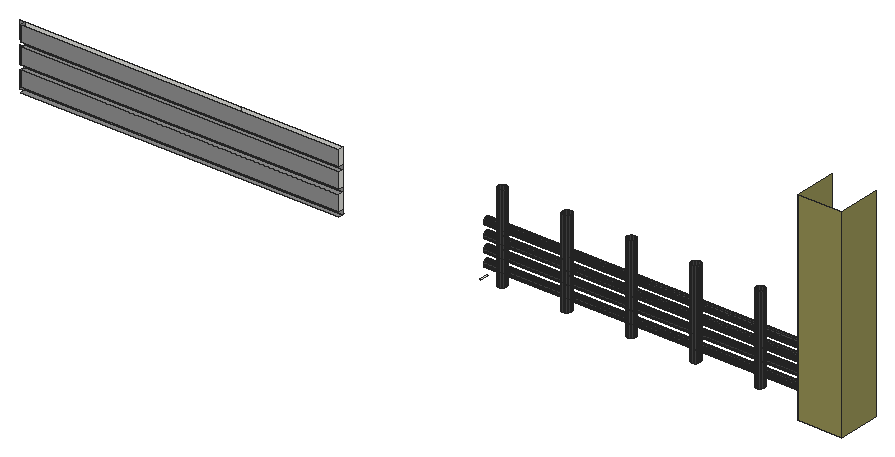
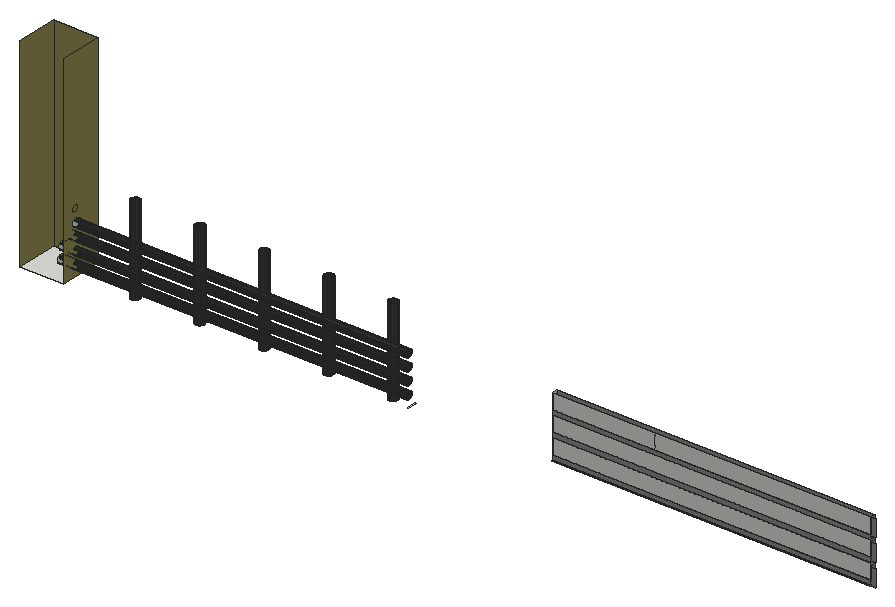
# SketchUp Ruby script. Lengths in inches.
U = 1.inch
M = Sketchup.active_model
def pt(a) = Geom::Point3d.new(a.map { |v| v * U })
def face(e, loops, mat)
  f = e.add_face(loops[0].map { |a| pt(a) })
  loops[1..].each { |l| e.add_face(l.map { |a| pt(a) }).erase! }
  f.material = f.back_material = mat if mat
  f
end
# faces: each face lists its corners as indices into pts; further lists are holes
def faces(e, pts, list, mat = nil) = list.each { |f| face(e, (f[0].is_a?(Array) ? f : [f]).map { |l| l.map { |i| pts[i] } }, mat) }
# xy, xz, yz: faces in a plane at the given z, y or x. An outline is a flat list of corners, or four numbers for a rectangle; further outlines are holes
def ring(l) = l.size == 4 ? [[l[0], l[1]], [l[2], l[1]], [l[2], l[3]], [l[0], l[3]]] : l.each_slice(2).to_a
def flat(e, list, mat, &to3) = list.each { |f| face(e, (f[0].is_a?(Array) ? f : [f]).map { |l| ring(l).map { |u, v| to3.(u, v) } }, mat) }
def xy(e, z, list, mat = nil) = flat(e, list, mat) { |x, y| [x, y, z] }
def xz(e, y, list, mat = nil) = flat(e, list, mat) { |x, z| [x, y, z] }
def yz(e, x, list, mat = nil) = flat(e, list, mat) { |y, z| [x, y, z] }
def lines(e, pts, list) = list.each { |a, b| e.add_line(pt(pts[a]), pt(pts[b])) }
# prism: a flat outline (further loops are holes) pulled along v
def prism(e, loops, v, mat = nil)
  f = face(e, loops, mat); d = Geom::Vector3d.new(v.map { |x| x * U })
  f.pushpull(f.normal.samedirection?(d) ? d.length : -d.length)
end
def box(e, o, s, mat = nil) = prism(e, [[o, [o[0] + s[0], o[1], o[2]], [o[0] + s[0], o[1] + s[1], o[2]], [o[0], o[1] + s[1], o[2]]]], [0, 0, s[2]], mat)
def at(x, y, z, deg = 0) = Geom::Transformation.translation(pt([x, y, z])) * Geom::Transformation.rotation(ORIGIN, Z_AXIS, deg.degrees)
def axes(o, x, y, z) = Geom::Transformation.new([*x, 0, *y, 0, *z, 0, *pt(o).to_a, 1])
def part(name) = M.definitions.add(name)
# library, detail: a bought-in or finely detailed component or shape, given as its bounding box
def library(name, o, s) = part(name).tap { |d| box(d.entities, o, s) }
def detail(e, o, s) = box(e.add_group.entities, o, s)
def put(e, d, t, mat = nil) = e.add_instance(d, t).tap { |i| i.material = mat if mat }
def group(e, t, mat = nil) = e.add_group.tap { |g| g.transformation = t; g.material = mat if mat }.entities
root = M.entities
M.materials.add("[0057_DarkKhaki]").color = [150, 145, 85]
M.materials.add("[0137_Black]").color = [71, 71, 71]
M.materials.add("[Color M05]").color = [145, 145, 145]
xy(root,379.43,[[[484.5625,1.0625,510.6875,26.4375],[488.89,12.9375,489.58,13.03,490.23,13.3,490.79,13.72,491.21,14.28,491.48,14.93,491.57,15.625,491.48,16.32,491.22,16.97,490.79,17.53,490.23,17.95,489.58,18.22,488.89,18.3125,488.19,18.22,487.54,17.95,486.99,17.53,486.56,16.97,486.29,16.32,486.2,15.625,486.29,14.93,486.56,14.28,486.99,13.73,487.54,13.3,488.19,13.03]],[488.89,12.9375,488.19,13.03,487.54,13.3,486.99,13.73,486.56,14.28,486.29,14.93,486.2,15.625,486.29,16.32,486.56,16.97,486.99,17.53,487.54,17.95,488.19,18.22,488.89,18.3125,489.58,18.22,490.23,17.95,490.79,17.53,491.22,16.97,491.48,16.32,491.57,15.625,491.48,14.93,491.21,14.28,490.79,13.72,490.23,13.3,489.58,13.03],[286.17,13.0625,286.99,18.1875]])
xy(root,381.65,[[11.875,18.1875,200.79,19]])
xy(root,381.65,[[11.875,15.1875,200.79,18.1875]],"[Color M05]")
xy(root,384.55,[[11.875,15.1875,200.79,18.1875]],"[Color M05]")
xy(root,393.65,[[11.875,15.1875,200.79,18.1875]],"[Color M05]")
xy(root,396.55,[[11.875,15.1875,200.79,18.1875]],"[Color M05]")
xy(root,405.65,[[11.875,15.1875,200.79,18.1875]],"[Color M05]")
xy(root,408.55,[[11.875,15.1875,200.79,18.1875]],"[Color M05]")
xz(root,1.0625,[[484.5625,379.43,510.6875,499.43]],"[0057_DarkKhaki]")
xz(root,15.1875,[[11.875,384.55,200.79,393.65],[11.875,396.55,200.79,405.65],[11.875,408.55,200.79,417.65]],"[Color M05]")
xz(root,18.1875,[[11.875,384.55,200.79,393.65],[11.875,396.55,200.79,405.65],[11.875,408.55,139.9375,417.65],[139.9375,408.55,200.79,417.65]])
xz(root,18.1875,[[8.875,381.32,11.875,391.4],[11.875,381.65,200.79,384.55],[11.875,393.65,200.79,396.55],[8.875,394.44,11.875,404.53],[11.875,405.65,200.79,408.55],
  [8.875,407.57,11.875,417.65]],"[Color M05]")
yz(root,11.875,[[18.1875,381.32,19,381.65]])
yz(root,11.875,[[15.1875,384.55,18.1875,391.4],[15.1875,391.4,18.1875,393.65],[15.1875,396.55,18.1875,404.53],[15.1875,404.53,18.1875,405.65],[15.1875,408.55,18.1875,417.65]],"[Color M05]")
yz(root,200.79,[[15.1875,384.55,18.1875,393.65],[15.1875,396.55,18.1875,405.65],[15.1875,408.55,18.1875,417.65]])
yz(root,484.11,[[18.04,406.36,18.63,406.44,19.17,406.66,19.64,407.02,19.99,407.49,20.22,408.03,20.29,408.61,20.22,409.2,19.99,409.74,19.64,410.2,19.17,410.5625,18.63,410.79,18.04,410.86,17.46,410.79,16.92,410.5625,16.45,410.2,16.1,409.74,15.87,409.2,15.79,408.61,15.87,408.03,16.1,407.49,16.45,407.02,16.92,406.66,17.46,406.44]])
yz(root,484.5625,[[[1.0625,379.43,26.4375,499.43],[18.04,413.86,18.63,413.94,19.17,414.16,19.64,414.52,19.99,414.99,20.22,415.53,20.29,416.11,20.22,416.7,19.99,417.24,19.64,417.7,19.17,418.0625,18.63,418.29,18.04,418.36,17.46,418.29,16.92,418.0625,16.45,417.7,16.1,417.24,15.87,416.7,15.79,416.11,15.87,415.53,16.1,414.99,16.45,414.52,16.92,414.16,17.46,413.94]]],"[0057_DarkKhaki]")
yz(root,487.23,[[18.04,398.86,18.63,398.94,19.17,399.16,19.64,399.52,19.99,399.99,20.22,400.53,20.29,401.11,20.22,401.7,19.99,402.24,19.64,402.7,19.17,403.0625,18.63,403.29,18.04,403.36,17.46,403.29,16.92,403.0625,16.45,402.7,16.1,402.24,15.87,401.7,15.79,401.11,15.87,400.53,16.1,399.99,16.45,399.52,16.92,399.16,17.46,398.94]])
yz(root,492.3,[[18.04,391.36,18.63,391.44,19.17,391.66,19.64,392.02,19.99,392.49,20.22,393.03,20.29,393.61,20.22,394.2,19.99,394.74,19.64,395.2,19.17,395.5625,18.63,395.79,18.04,395.86,17.46,395.79,16.92,395.5625,16.45,395.2,16.1,394.74,15.87,394.2,15.79,393.61,15.87,393.03,16.1,392.49,16.45,392.02,16.92,391.66,17.46,391.44]])
yz(root,492.98,[[18.04,383.86,18.63,383.94,19.17,384.16,19.64,384.52,19.99,384.99,20.22,385.53,20.29,386.11,20.22,386.7,19.99,387.24,19.64,387.7,19.17,388.0625,18.63,388.29,18.04,388.36,17.46,388.29,16.92,388.0625,16.45,387.7,16.1,387.24,15.87,386.7,15.79,386.11,15.87,385.53,16.1,384.99,16.45,384.52,16.92,384.16,17.46,383.94]])
yz(root,510.6875,[[1.0625,379.43,26.4375,499.43]],"[0057_DarkKhaki]")
p = [[296.94,13.03,379.43],[297.64,12.9375,379.43],[297.64,12.9375,431.18],[296.94,13.03,431.18],[298.33,13.03,379.43],[298.33,13.03,431.18],
  [335.19,13.03,379.43],[335.89,12.9375,379.43],[335.89,12.9375,431.18],[335.19,13.03,431.18],[336.58,13.03,379.43],[336.58,13.03,431.18],
  [373.44,13.03,379.43],[374.14,12.9375,379.43],[374.14,12.9375,431.18],[373.44,13.03,431.18],[374.83,13.03,379.43],[374.83,13.03,431.18],
  [411.69,13.03,379.43],[412.39,12.9375,379.43],[412.39,12.9375,431.18],[411.69,13.03,431.18],[413.08,13.03,379.43],[413.08,13.03,431.18],
  [449.94,13.03,379.43],[450.64,12.9375,379.43],[450.64,12.9375,431.18],[449.94,13.03,431.18],[451.33,13.03,379.43],[451.33,13.03,431.18],
  [296.29,13.3,379.43],[296.29,13.3,431.18],[298.98,13.3,379.43],[298.98,13.3,431.18],[334.54,13.3,379.43],[334.54,13.3,431.18],
  [337.23,13.3,379.43],[337.23,13.3,431.18],[372.79,13.3,379.43],[372.79,13.3,431.18],[375.48,13.3,379.43],[375.48,13.3,431.18],
  [411.04,13.3,379.43],[411.04,13.3,431.18],[413.73,13.3,379.43],[413.73,13.3,431.18],[449.29,13.3,379.43],[449.29,13.3,431.18],
  [451.98,13.3,379.43],[451.98,13.3,431.18],[295.74,13.73,379.43],[295.74,13.73,431.18],[299.54,13.72,379.43],[299.54,13.72,431.18],
  [333.99,13.73,379.43],[333.99,13.73,431.18],[337.79,13.72,379.43],[337.79,13.72,431.18],[372.24,13.73,379.43],[372.24,13.73,431.18],
  [376.04,13.72,379.43],[376.04,13.72,431.18],[410.49,13.73,379.43],[410.49,13.73,431.18],[414.29,13.72,379.43],[414.29,13.72,431.18],
  [448.74,13.73,379.43],[448.74,13.73,431.18],[452.54,13.72,379.43],[452.54,13.72,431.18],[295.31,14.28,379.43],[295.31,14.28,431.18],
  [299.96,14.28,379.43],[299.96,14.28,431.18],[333.56,14.28,379.43],[333.56,14.28,431.18],[338.21,14.28,379.43],[338.21,14.28,431.18],
  [371.81,14.28,379.43],[371.81,14.28,431.18],[376.46,14.28,379.43],[376.46,14.28,431.18],[410.06,14.28,379.43],[410.06,14.28,431.18],
  [414.71,14.28,379.43],[414.71,14.28,431.18],[448.31,14.28,379.43],[448.31,14.28,431.18],[452.96,14.28,379.43],[452.96,14.28,431.18],
  [295.04,14.93,379.43],[295.04,14.93,431.18],[300.23,14.93,379.43],[300.23,14.93,431.18],[333.29,14.93,379.43],[333.29,14.93,431.18],
  [338.48,14.93,379.43],[338.48,14.93,431.18],[371.54,14.93,379.43],[371.54,14.93,431.18],[376.73,14.93,379.43],[376.73,14.93,431.18],
  [409.79,14.93,379.43],[409.79,14.93,431.18],[414.98,14.93,379.43],[414.98,14.93,431.18],[448.04,14.93,379.43],[448.04,14.93,431.18],
  [453.23,14.93,379.43],[453.23,14.93,431.18],[294.95,15.625,379.43],[294.95,15.625,431.18],[300.32,15.625,379.43],[300.32,15.625,431.18],
  [333.2,15.625,379.43],[333.2,15.625,431.18],[338.57,15.625,379.43],[338.57,15.625,431.18],[371.45,15.625,379.43],[371.45,15.625,431.18],
  [376.82,15.625,379.43],[376.82,15.625,431.18],[409.7,15.625,379.43],[409.7,15.625,431.18],[415.07,15.625,379.43],[415.07,15.625,431.18],
  [447.95,15.625,379.43],[447.95,15.625,431.18],[453.32,15.625,379.43],[453.32,15.625,431.18],[295.04,16.32,379.43],[295.04,16.32,431.18],
  [300.23,16.32,379.43],[300.23,16.32,431.18],[333.29,16.32,379.43],[333.29,16.32,431.18],[338.48,16.32,379.43],[338.48,16.32,431.18],
  [371.54,16.32,379.43],[371.54,16.32,431.18],[376.73,16.32,379.43],[376.73,16.32,431.18],[409.79,16.32,379.43],[409.79,16.32,431.18],
  [414.98,16.32,379.43],[414.98,16.32,431.18],[448.04,16.32,379.43],[448.04,16.32,431.18],[453.23,16.32,379.43],[453.23,16.32,431.18],
  [295.31,16.97,379.43],[295.31,16.97,431.18],[299.97,16.97,379.43],[299.97,16.97,431.18],[333.56,16.97,379.43],[333.56,16.97,431.18],
  [338.22,16.97,379.43],[338.22,16.97,431.18],[371.81,16.97,379.43],[371.81,16.97,431.18],[376.47,16.97,379.43],[376.47,16.97,431.18],
  [410.06,16.97,379.43],[410.06,16.97,431.18],[414.72,16.97,379.43],[414.72,16.97,431.18],[448.31,16.97,379.43],[448.31,16.97,431.18],
  [452.97,16.97,379.43],[452.97,16.97,431.18],[295.74,17.53,379.43],[295.74,17.53,431.18],[299.54,17.53,379.43],[299.54,17.53,431.18],
  [333.99,17.53,379.43],[333.99,17.53,431.18],[337.79,17.53,379.43],[337.79,17.53,431.18],[372.24,17.53,379.43],[372.24,17.53,431.18],
  [376.04,17.53,379.43],[376.04,17.53,431.18],[410.49,17.53,379.43],[410.49,17.53,431.18],[414.29,17.53,379.43],[414.29,17.53,431.18],
  [448.74,17.53,379.43],[448.74,17.53,431.18],[452.54,17.53,379.43],[452.54,17.53,431.18],[296.29,17.95,379.43],[296.29,17.95,431.18],
  [298.98,17.95,379.43],[298.98,17.95,431.18],[334.54,17.95,379.43],[334.54,17.95,431.18],[337.23,17.95,379.43],[337.23,17.95,431.18],
  [372.79,17.95,379.43],[372.79,17.95,431.18],[375.48,17.95,379.43],[375.48,17.95,431.18],[411.04,17.95,379.43],[411.04,17.95,431.18],
  [413.73,17.95,379.43],[413.73,17.95,431.18],[449.29,17.95,379.43],[449.29,17.95,431.18],[451.98,17.95,379.43],[451.98,17.95,431.18],
  [296.94,18.22,379.43],[296.94,18.22,431.18],[298.33,18.22,379.43],[298.33,18.22,431.18],[335.19,18.22,379.43],[335.19,18.22,431.18],
  [336.58,18.22,379.43],[336.58,18.22,431.18],[373.44,18.22,379.43],[373.44,18.22,431.18],[374.83,18.22,379.43],[374.83,18.22,431.18],
  [411.69,18.22,379.43],[411.69,18.22,431.18],[413.08,18.22,379.43],[413.08,18.22,431.18],[449.94,18.22,379.43],[449.94,18.22,431.18],
  [451.33,18.22,379.43],[451.33,18.22,431.18],[297.64,18.3125,379.43],[297.64,18.3125,431.18],[335.89,18.3125,379.43],[335.89,18.3125,431.18],
  [374.14,18.3125,379.43],[374.14,18.3125,431.18],[412.39,18.3125,379.43],[412.39,18.3125,431.18],[450.64,18.3125,379.43],[450.64,18.3125,431.18],
  [286.17,16.92,384.16],[286.17,17.46,383.94],[492.98,17.46,383.94],[492.98,16.92,384.16],[286.17,18.04,383.86],[492.98,18.04,383.86],
  [286.17,18.63,383.94],[492.98,18.63,383.94],[286.17,19.17,384.16],[492.98,19.17,384.16],[286.17,16.45,384.52],[492.98,16.45,384.52],
  [286.17,19.64,384.52],[492.98,19.64,384.52],[286.17,16.1,384.99],[492.98,16.1,384.99],[286.17,19.99,384.99],[492.98,19.99,384.99],
  [286.17,15.87,385.53],[492.98,15.87,385.53],[286.17,15.79,386.11],[492.98,15.79,386.11],[286.17,15.87,386.7],[492.98,15.87,386.7],
  [286.17,16.1,387.24],[492.98,16.1,387.24],[286.17,16.45,387.7],[492.98,16.45,387.7],[286.17,19.99,387.24],[286.17,19.64,387.7],
  [492.98,19.64,387.7],[492.98,19.99,387.24],[286.17,16.92,388.0625],[492.98,16.92,388.0625],[286.17,19.17,388.0625],[492.98,19.17,388.0625],
  [286.17,17.46,388.29],[492.98,17.46,388.29],[286.17,18.63,388.29],[492.98,18.63,388.29],[286.17,18.04,388.36],[492.98,18.04,388.36],
  [286.17,16.92,391.66],[286.17,17.46,391.44],[492.3,17.46,391.44],[492.3,16.92,391.66],[286.17,18.04,391.36],[492.3,18.04,391.36],
  [286.17,18.63,391.44],[492.3,18.63,391.44],[286.17,19.17,391.66],[492.3,19.17,391.66],[286.17,16.45,392.02],[492.3,16.45,392.02],
  [286.17,19.64,392.02],[492.3,19.64,392.02],[286.17,16.1,392.49],[492.3,16.1,392.49],[286.17,19.99,392.49],[492.3,19.99,392.49],
  [286.17,15.87,393.03],[492.3,15.87,393.03],[286.17,15.79,393.61],[492.3,15.79,393.61],[286.17,15.87,394.2],[492.3,15.87,394.2],
  [286.17,16.1,394.74],[492.3,16.1,394.74],[286.17,16.45,395.2],[492.3,16.45,395.2],[286.17,16.92,395.5625],[492.3,16.92,395.5625],
  [286.17,19.64,395.2],[286.17,19.17,395.5625],[492.3,19.17,395.5625],[492.3,19.64,395.2],[286.17,17.46,395.79],[492.3,17.46,395.79],
  [286.17,18.63,395.79],[492.3,18.63,395.79],[286.17,18.04,395.86],[492.3,18.04,395.86],[286.17,16.92,399.16],[286.17,17.46,398.94],
  [487.23,17.46,398.94],[487.23,16.92,399.16],[286.17,18.04,398.86],[487.23,18.04,398.86],[286.17,18.63,398.94],[487.23,18.63,398.94],
  [286.17,19.17,399.16],[487.23,19.17,399.16],[286.17,16.45,399.52],[487.23,16.45,399.52],[286.17,19.64,399.52],[487.23,19.64,399.52],
  [286.17,16.1,399.99],[487.23,16.1,399.99],[286.17,15.87,400.53],[487.23,15.87,400.53],[286.17,15.79,401.11],[487.23,15.79,401.11],
  [286.17,15.87,401.7],[487.23,15.87,401.7],[286.17,16.1,402.24],[487.23,16.1,402.24],[286.17,16.45,402.7],[487.23,16.45,402.7],
  [286.17,16.92,403.0625],[487.23,16.92,403.0625],[286.17,19.64,402.7],[286.17,19.17,403.0625],[487.23,19.17,403.0625],[487.23,19.64,402.7],
  [286.17,17.46,403.29],[487.23,17.46,403.29],[286.17,18.63,403.29],[487.23,18.63,403.29],[286.17,18.04,403.36],[487.23,18.04,403.36],
  [286.17,16.92,406.66],[286.17,17.46,406.44],[484.11,17.46,406.44],[484.11,16.92,406.66],[286.17,18.04,406.36],[484.11,18.04,406.36],
  [286.17,18.63,406.44],[484.11,18.63,406.44],[286.17,19.17,406.66],[484.11,19.17,406.66],[286.17,16.45,407.02],[484.11,16.45,407.02],
  [286.17,19.64,407.02],[484.11,19.64,407.02],[286.17,16.1,407.49],[484.11,16.1,407.49],[286.17,15.87,408.03],[484.11,15.87,408.03],
  [286.17,15.79,408.61],[484.11,15.79,408.61],[286.17,15.87,409.2],[484.11,15.87,409.2],[286.17,16.1,409.74],[484.11,16.1,409.74],
  [286.17,16.45,410.2],[484.11,16.45,410.2],[286.17,16.92,410.5625],[484.11,16.92,410.5625],[286.17,19.64,410.2],[286.17,19.17,410.5625],
  [484.11,19.17,410.5625],[484.11,19.64,410.2],[286.17,17.46,410.79],[484.11,17.46,410.79],[286.17,18.63,410.79],[484.11,18.63,410.79],
  [286.17,18.04,410.86],[484.11,18.04,410.86],[284.41,1.0625,379.43],[284.05,1.0625,379.43],[285.29,1.0625,379.43],[286.99,1.0625,379.43],
  [11.875,19,381.65],[8.875,19,381.65]]
faces(root,p,[[0,1,2,3],[1,4,5,2],[6,7,8,9],[7,10,11,8],[12,13,14,15],[13,16,17,14],[18,19,20,21],[19,22,23,20],
  [24,25,26,27],[25,28,29,26],[30,0,3,31],[4,32,33,5],[34,6,9,35],[10,36,37,11],[38,12,15,39],[16,40,41,17],
  [42,18,21,43],[22,44,45,23],[46,24,27,47],[28,48,49,29],[50,30,31,51],[32,52,53,33],[54,34,35,55],[36,56,57,37],
  [58,38,39,59],[40,60,61,41],[62,42,43,63],[44,64,65,45],[66,46,47,67],[48,68,69,49],[70,50,51,71],[52,72,73,53],
  [74,54,55,75],[56,76,77,57],[78,58,59,79],[60,80,81,61],[82,62,63,83],[64,84,85,65],[86,66,67,87],[68,88,89,69],
  [90,70,71,91],[72,92,93,73],[94,74,75,95],[76,96,97,77],[98,78,79,99],[80,100,101,81],[102,82,83,103],[84,104,105,85],
  [106,86,87,107],[88,108,109,89],[110,90,91,111],[92,112,113,93],[114,94,95,115],[96,116,117,97],[118,98,99,119],[100,120,121,101],
  [122,102,103,123],[104,124,125,105],[126,106,107,127],[108,128,129,109],[130,110,111,131],[112,132,133,113],[134,114,115,135],[116,136,137,117],
  [138,118,119,139],[120,140,141,121],[142,122,123,143],[124,144,145,125],[146,126,127,147],[128,148,149,129],[150,130,131,151],[132,152,153,133],
  [154,134,135,155],[136,156,157,137],[158,138,139,159],[140,160,161,141],[162,142,143,163],[144,164,165,145],[166,146,147,167],[148,168,169,149],
  [170,150,151,171],[152,172,173,153],[174,154,155,175],[156,176,177,157],[178,158,159,179],[160,180,181,161],[182,162,163,183],[164,184,185,165],
  [186,166,167,187],[168,188,189,169],[190,170,171,191],[172,192,193,173],[194,174,175,195],[176,196,197,177],[198,178,179,199],[180,200,201,181],
  [202,182,183,203],[184,204,205,185],[206,186,187,207],[188,208,209,189],[210,190,191,211],[192,212,213,193],[214,194,195,215],[196,216,217,197],
  [218,198,199,219],[200,220,221,201],[222,202,203,223],[204,224,225,205],[226,206,207,227],[208,228,229,209],[230,210,211,231],[212,230,231,213],
  [232,214,215,233],[216,232,233,217],[234,218,219,235],[220,234,235,221],[236,222,223,237],[224,236,237,225],[238,226,227,239],[228,238,239,229],
  [240,241,242,243],[241,244,245,242],[244,246,247,245],[246,248,249,247],[250,240,243,251],[248,252,253,249],[254,250,251,255],[252,256,257,253],
  [258,254,255,259],[260,258,259,261],[262,260,261,263],[264,262,263,265],[266,264,265,267],[268,269,270,271],[272,266,267,273],[269,274,275,270],
  [276,272,273,277],[274,278,279,275],[280,276,277,281],[278,280,281,279],[282,283,284,285],[283,286,287,284],[286,288,289,287],[288,290,291,289],
  [292,282,285,293],[290,294,295,291],[296,292,293,297],[294,298,299,295],[300,296,297,301],[302,300,301,303],[304,302,303,305],[306,304,305,307],
  [308,306,307,309],[310,308,309,311],[312,313,314,315],[316,310,311,317],[313,318,319,314],[320,316,317,321],[318,320,321,319],[322,323,324,325],
  [323,326,327,324],[326,328,329,327],[328,330,331,329],[332,322,325,333],[330,334,335,331],[336,332,333,337],[338,336,337,339],[340,338,339,341],
  [342,340,341,343],[344,342,343,345],[346,344,345,347],[348,346,347,349],[350,351,352,353],[354,348,349,355],[351,356,357,352],[358,354,355,359],
  [356,358,359,357],[360,361,362,363],[361,364,365,362],[364,366,367,365],[366,368,369,367],[370,360,363,371],[368,372,373,369],[374,370,371,375],
  [376,374,375,377],[378,376,377,379],[380,378,379,381],[382,380,381,383],[384,382,383,385],[386,384,385,387],[388,389,390,391],[392,386,387,393],
  [389,394,395,390],[396,392,393,397],[394,396,397,395]],"[0137_Black]")
lines(root,p,[[398,399],[400,401],[402,403]])
